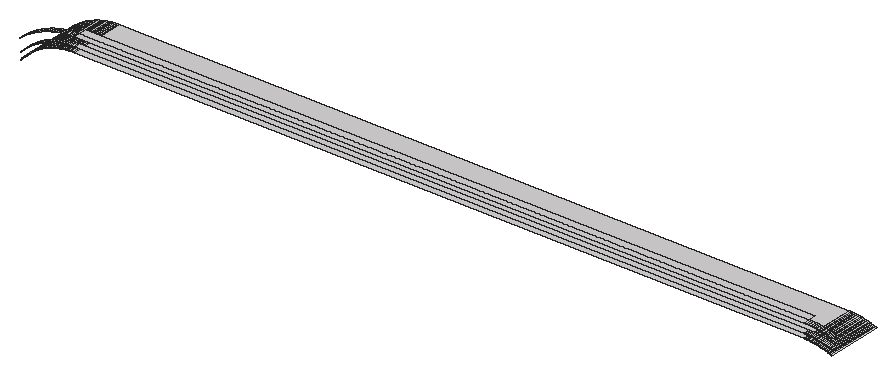
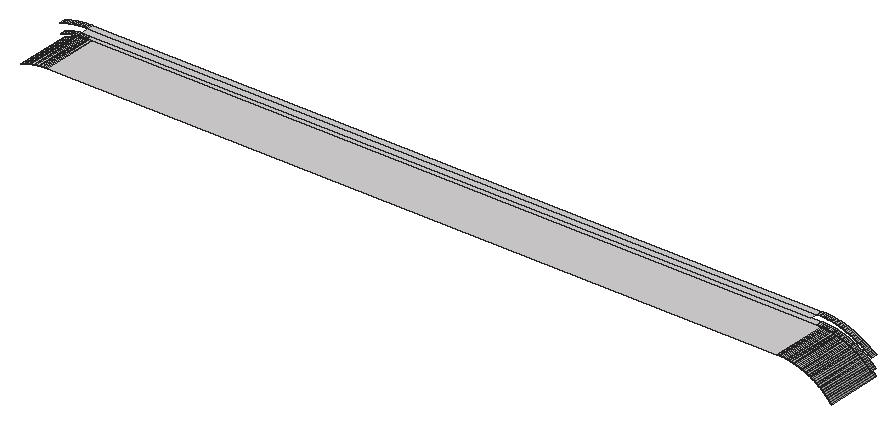
# SketchUp Ruby script. Lengths in inches.
U = 1.inch
M = Sketchup.active_model
def pt(a) = Geom::Point3d.new(a.map { |v| v * U })
def face(e, loops, mat)
  f = e.add_face(loops[0].map { |a| pt(a) })
  loops[1..].each { |l| e.add_face(l.map { |a| pt(a) }).erase! }
  f.material = f.back_material = mat if mat
  f
end
# faces: each face lists its corners as indices into pts; further lists are holes
def faces(e, pts, list, mat = nil) = list.each { |f| face(e, (f[0].is_a?(Array) ? f : [f]).map { |l| l.map { |i| pts[i] } }, mat) }
# xy, xz, yz: faces in a plane at the given z, y or x. An outline is a flat list of corners, or four numbers for a rectangle; further outlines are holes
def ring(l) = l.size == 4 ? [[l[0], l[1]], [l[2], l[1]], [l[2], l[3]], [l[0], l[3]]] : l.each_slice(2).to_a
def flat(e, list, mat, &to3) = list.each { |f| face(e, (f[0].is_a?(Array) ? f : [f]).map { |l| ring(l).map { |u, v| to3.(u, v) } }, mat) }
def xy(e, z, list, mat = nil) = flat(e, list, mat) { |x, y| [x, y, z] }
def xz(e, y, list, mat = nil) = flat(e, list, mat) { |x, z| [x, y, z] }
def yz(e, x, list, mat = nil) = flat(e, list, mat) { |y, z| [x, y, z] }
def lines(e, pts, list) = list.each { |a, b| e.add_line(pt(pts[a]), pt(pts[b])) }
# prism: a flat outline (further loops are holes) pulled along v
def prism(e, loops, v, mat = nil)
  f = face(e, loops, mat); d = Geom::Vector3d.new(v.map { |x| x * U })
  f.pushpull(f.normal.samedirection?(d) ? d.length : -d.length)
end
def box(e, o, s, mat = nil) = prism(e, [[o, [o[0] + s[0], o[1], o[2]], [o[0] + s[0], o[1] + s[1], o[2]], [o[0], o[1] + s[1], o[2]]]], [0, 0, s[2]], mat)
def at(x, y, z, deg = 0) = Geom::Transformation.translation(pt([x, y, z])) * Geom::Transformation.rotation(ORIGIN, Z_AXIS, deg.degrees)
def axes(o, x, y, z) = Geom::Transformation.new([*x, 0, *y, 0, *z, 0, *pt(o).to_a, 1])
def part(name) = M.definitions.add(name)
# library, detail: a bought-in or finely detailed component or shape, given as its bounding box
def library(name, o, s) = part(name).tap { |d| box(d.entities, o, s) }
def detail(e, o, s) = box(e.add_group.entities, o, s)
def put(e, d, t, mat = nil) = e.add_instance(d, t).tap { |i| i.material = mat if mat }
def group(e, t, mat = nil) = e.add_group.tap { |g| g.transformation = t; g.material = mat if mat }.entities
root = M.entities
M.materials.add("[Quartz Light Brown]").color = [215, 212, 212]
xy(root,350.99,[[292.91,143,293.11,155],[450.39,143,450.59,155]],"[Quartz Light Brown]")
xy(root,351,[[293.3,143,293.5,155],[293.5,143,450,155],[450,143,450.2,155]],"[Quartz Light Brown]")
xy(root,351.99,[[292.87,143,293.08,144.25],[450.42,143,450.63,144.25]],"[Quartz Light Brown]")
xy(root,352,[[293.29,143,293.5,144.25],[293.5,143,450,144.25],[450,143,450.21,144.25]],"[Quartz Light Brown]")
xy(root,353.99,[[292.79,143,293.03,144.25],[450.47,143,450.71,144.25]],"[Quartz Light Brown]")
xy(root,354,[[293.26,143,293.5,144.25],[293.5,143,450,144.25],[450,143,450.24,144.25],[293.5,144.25,450,146]],"[Quartz Light Brown]")
p = [[281.97,143,345.59],[281.84,143,345.44],[281.84,155,345.44],[281.97,155,345.59],[282.09,143,345.74],[282.09,155,345.74],
  [282.22,143,345.89],[282.22,155,345.89],[282.35,143,346.04],[282.35,155,346.04],[282.49,143,346.18],[282.49,155,346.18],
  [282.62,143,346.33],[282.62,155,346.33],[282.76,143,346.47],[282.76,155,346.47],[282.89,143,346.61],[282.89,155,346.61],
  [283.03,143,346.74],[283.03,155,346.74],[283.17,143,346.88],[283.17,155,346.88],[283.32,143,347.01],[283.32,155,347.01],
  [281.89,143,347.01],[282.04,143,347.16],[282.04,144.25,347.16],[281.89,144.25,347.01],[283.46,143,347.15],[283.46,155,347.15],
  [283.61,143,347.28],[283.61,155,347.28],[282.1875,143,347.3125],[282.1875,144.25,347.3125],[282.34,143,347.46],[282.34,144.25,347.46],
  [283.76,143,347.41],[283.76,155,347.41],[283.91,143,347.53],[283.91,155,347.53],[282.49,143,347.61],[282.49,144.25,347.61],
  [284.06,143,347.66],[284.06,155,347.66],[282.64,143,347.75],[282.64,144.25,347.75],[282.79,143,347.89],[282.79,144.25,347.89],
  [284.21,143,347.78],[284.21,155,347.78],[284.37,143,347.9],[284.37,155,347.9],[282.95,143,348.03],[282.95,144.25,348.03],
  [284.53,143,348.02],[284.53,155,348.02],[283.11,143,348.17],[283.11,144.25,348.17],[284.68,143,348.14],[284.68,155,348.14],
  [284.84,143,348.25],[284.84,155,348.25],[283.27,143,348.3],[283.27,144.25,348.3],[285,143,348.36],[285,155,348.36],
  [283.43,143,348.43],[283.43,144.25,348.43],[283.59,143,348.57],[283.59,144.25,348.57],[285.17,143,348.47],[285.17,155,348.47],
  [285.33,143,348.58],[285.33,155,348.58],[283.76,143,348.69],[283.76,144.25,348.69],[285.5,143,348.6875],[285.5,155,348.6875],
  [283.93,143,348.82],[283.93,144.25,348.82],[285.66,143,348.79],[285.66,155,348.79],[284.1,143,348.94],[284.1,144.25,348.94],
  [285.83,143,348.89],[285.83,155,348.89],[284.27,143,349.07],[284.27,144.25,349.07],[286,143,348.99],[286,155,348.99],
  [286.17,143,349.09],[286.17,155,349.09],[284.4375,143,349.1875],[284.4375,144.25,349.1875],[286.34,143,349.18],[286.34,155,349.18],
  [284.61,143,349.3],[284.61,144.25,349.3],[286.52,143,349.27],[286.52,155,349.27],[284.79,143,349.42],[284.79,144.25,349.42],
  [286.69,143,349.37],[286.69,155,349.37],[284.96,143,349.53],[284.96,144.25,349.53],[286.87,143,349.45],[286.87,155,349.45],
  [285.14,143,349.64],[285.14,144.25,349.64],[287.04,143,349.54],[287.04,155,349.54],[287.22,143,349.62],[287.22,155,349.62],
  [285.32,143,349.75],[285.32,144.25,349.75],[287.4,143,349.7],[287.4,155,349.7],[281.99,144.25,349.84],[281.99,143,349.84],
  [281.81,143,349.6875],[281.81,144.25,349.6875],[287.58,143,349.78],[287.58,155,349.78],[282.17,144.25,349.99],[282.17,143,349.99],
  [285.5,143,349.86],[285.5,144.25,349.86],[287.76,143,349.86],[287.76,155,349.86],[455.92,143,349.78],[455.74,143,349.86],
  [455.74,155,349.86],[455.92,155,349.78],[285.68,143,349.96],[285.68,144.25,349.96],[287.94,143,349.93],[287.94,155,349.93],
  [288.125,143,350],[288.125,155,350],[455.56,143,349.93],[455.375,143,350],[455.375,155,350],[455.56,155,349.93],
  [282.36,144.25,350.14],[282.36,143,350.14],[285.87,143,350.0625],[285.87,144.25,350.0625],[288.31,143,350.07],[288.31,155,350.07],
  [455.19,143,350.07],[455.19,155,350.07],[282.54,144.25,350.28],[282.54,143,350.28],[286.05,143,350.16],[286.05,144.25,350.16],
  [288.49,143,350.14],[288.49,155,350.14],[288.68,143,350.2],[288.68,155,350.2],[455.01,143,350.14],[454.82,143,350.2],
  [454.82,155,350.2],[455.01,155,350.14],[286.24,143,350.26],[286.24,144.25,350.26],[288.86,143,350.27],[288.86,155,350.27],
  [454.64,143,350.27],[454.64,155,350.27],[282.73,144.25,350.42],[282.73,143,350.42],[286.42,143,350.35],[286.42,144.25,350.35],
  [286.61,143,350.44],[286.61,144.25,350.44],[289.05,143,350.33],[289.05,155,350.33],[289.24,143,350.38],[289.24,155,350.38],
  [454.45,143,350.33],[454.26,143,350.38],[454.26,155,350.38],[454.45,155,350.33],[282.92,144.25,350.5625],[282.92,143,350.5625],
  [286.8,143,350.53],[286.8,144.25,350.53],[289.43,143,350.4375],[289.43,155,350.4375],[289.62,143,350.49],[289.62,155,350.49],
  [454.07,143,350.4375],[453.88,143,350.49],[453.88,155,350.49],[454.07,155,350.4375],[286.99,143,350.62],[286.99,144.25,350.62],
  [289.81,143,350.54],[289.81,155,350.54],[290,143,350.59],[290,155,350.59],[453.69,143,350.54],[453.5,143,350.59],
  [453.5,155,350.59],[453.69,155,350.54],[283.11,144.25,350.7],[283.11,143,350.7],[287.18,143,350.7],[287.18,144.25,350.7],
  [290.19,143,350.63],[290.19,155,350.63],[290.38,143,350.67],[290.38,155,350.67],[453.31,143,350.63],[453.12,143,350.67],
  [453.12,155,350.67],[453.31,155,350.63],[283.3,144.25,350.83],[283.3,143,350.83],[287.38,143,350.78],[287.38,144.25,350.78],
  [290.57,143,350.71],[290.57,155,350.71],[290.77,143,350.75],[290.77,155,350.75],[290.96,143,350.78],[290.96,155,350.78],
  [452.73,143,350.75],[452.54,143,350.78],[452.54,155,350.78],[452.73,155,350.75],[452.93,143,350.71],[452.93,155,350.71],
  [283.5,144.25,350.97],[283.5,143,350.97],[287.57,143,350.86],[287.57,144.25,350.86],[291.15,143,350.82],[291.15,155,350.82],
  [291.35,143,350.84],[291.35,155,350.84],[291.54,143,350.87],[291.54,155,350.87],[452.15,143,350.84],[451.96,143,350.87],
  [451.96,155,350.87],[452.15,155,350.84],[452.35,143,350.82],[452.35,155,350.82],[287.77,143,350.9375],[287.77,144.25,350.9375],
  [287.96,143,351.01],[287.96,144.25,351.01],[291.74,143,350.9],[291.74,155,350.9],[291.93,143,350.92],[291.93,155,350.92],
  [292.13,143,350.9375],[292.13,155,350.9375],[292.32,143,350.95],[292.32,155,350.95],[451.37,143,350.9375],[451.18,143,350.95],
  [451.18,155,350.95],[451.37,155,350.9375],[451.57,143,350.92],[451.57,155,350.92],[451.76,143,350.9],[451.76,155,350.9],
  [455.54,143,351.01],[455.73,143,350.9375],[455.73,144.25,350.9375],[455.54,144.25,351.01],[455.93,143,350.86],[455.93,144.25,350.86],
  [283.7,144.25,351.1],[283.7,143,351.1],[288.16,143,351.08],[288.16,144.25,351.08],[292.52,143,350.97],[292.52,155,350.97],
  [292.71,143,350.98],[292.71,155,350.98],[292.91,143,350.99],[292.91,155,350.99],[293.3,143,351],[293.11,143,350.99],
  [293.11,155,350.99],[293.3,155,351],[450.39,143,350.99],[450.2,143,351],[450.2,155,351],[450.39,155,350.99],
  [450.79,143,350.98],[450.59,143,350.99],[450.59,155,350.99],[450.79,155,350.98],[450.98,143,350.97],[450.98,155,350.97],
  [455.34,143,351.08],[455.34,144.25,351.08],[283.89,144.25,351.22],[283.89,143,351.22],[288.36,143,351.15],[288.36,144.25,351.15],
  [455.14,143,351.15],[455.14,144.25,351.15],[284.1,144.25,351.35],[284.1,143,351.35],[288.56,143,351.22],[288.56,144.25,351.22],
  [288.76,143,351.28],[288.76,144.25,351.28],[454.74,143,351.28],[454.94,143,351.22],[454.94,144.25,351.22],[454.74,144.25,351.28],
  [284.3,144.25,351.47],[284.3,143,351.47],[288.96,143,351.34],[288.96,144.25,351.34],[289.16,143,351.4],[289.16,144.25,351.4],
  [454.34,143,351.4],[454.54,143,351.34],[454.54,144.25,351.34],[454.34,144.25,351.4],[289.36,143,351.45],[289.36,144.25,351.45],
  [454.14,143,351.45],[454.14,144.25,351.45],[284.5,144.25,351.59],[284.5,143,351.59],[289.5625,143,351.51],[289.5625,144.25,351.51],
  [289.76,143,351.56],[289.76,144.25,351.56],[453.74,143,351.56],[453.9375,143,351.51],[453.9375,144.25,351.51],[453.74,144.25,351.56],
  [284.7,144.25,351.7],[284.7,143,351.7],[289.97,143,351.61],[289.97,144.25,351.61],[290.17,143,351.65],[290.17,144.25,351.65],
  [453.33,143,351.65],[453.53,143,351.61],[453.53,144.25,351.61],[453.33,144.25,351.65],[284.91,144.25,351.82],[284.91,143,351.82],
  [290.38,143,351.69],[290.38,144.25,351.69],[290.58,143,351.73],[290.58,144.25,351.73],[290.79,143,351.77],[290.79,144.25,351.77],
  [452.71,143,351.77],[452.92,143,351.73],[452.92,144.25,351.73],[452.71,144.25,351.77],[453.12,143,351.69],[453.12,144.25,351.69],
  [285.12,144.25,351.93],[285.12,143,351.93],[291,143,351.8],[291,144.25,351.8],[291.2,143,351.83],[291.2,144.25,351.83],
  [291.41,143,351.86],[291.41,144.25,351.86],[452.09,143,351.86],[452.3,143,351.83],[452.3,144.25,351.83],[452.09,144.25,351.86],
  [452.5,143,351.8],[452.5,144.25,351.8],[285.33,144.25,352.04],[285.33,143,352.04],[291.62,143,351.89],[291.62,144.25,351.89],
  [291.83,143,351.91],[291.83,144.25,351.91],[292.04,143,351.93],[292.04,144.25,351.93],[292.24,143,351.95],[292.24,144.25,351.95],
  [451.26,143,351.95],[451.46,143,351.93],[451.46,144.25,351.93],[451.26,144.25,351.95],[451.67,143,351.91],[451.67,144.25,351.91],
  [451.88,143,351.89],[451.88,144.25,351.89],[285.54,144.25,352.14],[285.54,143,352.14],[292.45,143,351.97],[292.45,144.25,351.97],
  [292.66,143,351.98],[292.66,144.25,351.98],[292.87,143,351.99],[292.87,144.25,351.99],[293.08,143,351.99],[293.29,143,352],
  [293.29,144.25,352],[293.08,144.25,351.99],[450.21,143,352],[450.42,143,351.99],[450.42,144.25,351.99],[450.21,144.25,352],
  [450.63,143,351.99],[450.84,143,351.98],[450.84,144.25,351.98],[450.63,144.25,351.99],[451.05,143,351.97],[451.05,144.25,351.97],
  [285.75,144.25,352.25],[285.75,143,352.25],[285.96,144.25,352.35],[285.96,143,352.35],[286.18,144.25,352.44],[286.18,143,352.44],
  [286.39,144.25,352.54],[286.39,143,352.54],[286.61,144.25,352.63],[286.61,143,352.63],[286.83,144.25,352.72],[286.83,143,352.72],
  [287.05,144.25,352.8],[287.05,143,352.8],[287.27,144.25,352.89],[287.27,143,352.89],[287.49,144.25,352.97],[287.49,143,352.97],
  [287.71,144.25,353.04],[287.71,143,353.04],[287.9375,144.25,353.12],[287.9375,143,353.12],[455.79,144.25,353.04],[455.79,143,353.04],
  [455.5625,143,353.12],[455.5625,144.25,353.12],[456.01,144.25,352.97],[456.01,143,352.97],[288.16,144.25,353.19],[288.16,143,353.19],
  [455.34,143,353.19],[455.34,144.25,353.19],[288.39,144.25,353.26],[288.39,143,353.26],[455.11,143,353.26],[455.11,144.25,353.26],
  [288.61,144.25,353.32],[288.61,143,353.32],[288.84,144.25,353.39],[288.84,143,353.39],[454.89,144.25,353.32],[454.89,143,353.32],
  [454.66,143,353.39],[454.66,144.25,353.39],[289.07,144.25,353.45],[289.07,143,353.45],[289.3,144.25,353.5],[289.3,143,353.5],
  [454.43,144.25,353.45],[454.43,143,353.45],[454.2,143,353.5],[454.2,144.25,353.5],[289.53,144.25,353.56],[289.53,143,353.56],
  [453.97,143,353.56],[453.97,144.25,353.56],[289.76,144.25,353.61],[289.76,143,353.61],[289.99,144.25,353.65],[289.99,143,353.65],
  [453.74,144.25,353.61],[453.74,143,353.61],[453.51,143,353.65],[453.51,144.25,353.65],[290.22,144.25,353.7],[290.22,143,353.7],
  [290.45,144.25,353.74],[290.45,143,353.74],[290.68,144.25,353.78],[290.68,143,353.78],[453.05,144.25,353.74],[453.05,143,353.74],
  [452.82,143,353.78],[452.82,144.25,353.78],[453.28,144.25,353.7],[453.28,143,353.7],[290.92,144.25,353.8125],[290.92,143,353.8125],
  [291.15,144.25,353.85],[291.15,143,353.85],[291.38,144.25,353.875],[291.38,143,353.875],[452.35,144.25,353.85],[452.35,143,353.85],
  [452.12,143,353.875],[452.12,144.25,353.875],[452.58,144.25,353.8125],[452.58,143,353.8125],[291.62,144.25,353.9],[291.62,143,353.9],
  [291.85,144.25,353.92],[291.85,143,353.92],[292.09,144.25,353.94],[292.09,143,353.94],[292.32,144.25,353.96],[292.32,143,353.96],
  [451.41,144.25,353.94],[451.41,143,353.94],[451.18,143,353.96],[451.18,144.25,353.96],[451.65,144.25,353.92],[451.65,143,353.92],
  [451.88,144.25,353.9],[451.88,143,353.9],[292.56,144.25,353.98],[292.56,143,353.98],[292.79,144.25,353.99],[292.79,143,353.99],
  [293.26,144.25,354],[293.26,143,354],[293.03,143,353.99],[293.03,144.25,353.99],[450.47,144.25,353.99],[450.47,143,353.99],
  [450.24,143,354],[450.24,144.25,354],[450.94,144.25,353.98],[450.94,143,353.98],[450.71,143,353.99],[450.71,144.25,353.99]]
faces(root,p,[[0,1,2,3],[4,0,3,5],[6,4,5,7],[8,6,7,9],[10,8,9,11],[12,10,11,13],[14,12,13,15],[16,14,15,17],
  [18,16,17,19],[20,18,19,21],[22,20,21,23],[24,25,26,27],[28,22,23,29],[30,28,29,31],[25,32,33,26],[32,34,35,33],
  [36,30,31,37],[38,36,37,39],[34,40,41,35],[42,38,39,43],[40,44,45,41],[44,46,47,45],[48,42,43,49],[50,48,49,51],
  [46,52,53,47],[54,50,51,55],[52,56,57,53],[58,54,55,59],[60,58,59,61],[56,62,63,57],[64,60,61,65],[62,66,67,63],
  [66,68,69,67],[70,64,65,71],[72,70,71,73],[68,74,75,69],[76,72,73,77],[74,78,79,75],[80,76,77,81],[78,82,83,79],
  [84,80,81,85],[82,86,87,83],[88,84,85,89],[90,88,89,91],[86,92,93,87],[94,90,91,95],[92,96,97,93],[98,94,95,99],
  [96,100,101,97],[102,98,99,103],[100,104,105,101],[106,102,103,107],[104,108,109,105],[110,106,107,111],[112,110,111,113],[108,114,115,109],
  [116,112,113,117],[118,119,120,121],[122,116,117,123],[124,125,119,118],[114,126,127,115],[128,122,123,129],[130,131,132,133],[126,134,135,127],
  [136,128,129,137],[138,136,137,139],[140,141,142,143],[131,140,143,132],[144,145,125,124],[134,146,147,135],[148,138,139,149],[141,150,151,142],
  [152,153,145,144],[146,154,155,147],[156,148,149,157],[158,156,157,159],[160,161,162,163],[150,160,163,151],[154,164,165,155],[166,158,159,167],
  [161,168,169,162],[170,171,153,152],[164,172,173,165],[172,174,175,173],[176,166,167,177],[178,176,177,179],[180,181,182,183],[168,180,183,169],
  [184,185,171,170],[174,186,187,175],[188,178,179,189],[190,188,189,191],[192,193,194,195],[181,192,195,182],[186,196,197,187],[198,190,191,199],
  [200,198,199,201],[202,203,204,205],[193,202,205,194],[206,207,185,184],[196,208,209,197],[210,200,201,211],[212,210,211,213],[214,215,216,217],
  [203,214,217,204],[218,219,207,206],[208,220,221,209],[222,212,213,223],[224,222,223,225],[226,224,225,227],[228,229,230,231],[232,228,231,233],
  [215,232,233,216],[234,235,219,218],[220,236,237,221],[238,226,227,239],[240,238,239,241],[242,240,241,243],[244,245,246,247],[248,244,247,249],
  [229,248,249,230],[236,250,251,237],[250,252,253,251],[254,242,243,255],[256,254,255,257],[258,256,257,259],[260,258,259,261],[262,263,264,265],
  [266,262,265,267],[268,266,267,269],[245,268,269,246],[270,271,272,273],[271,274,275,272],[276,277,235,234],[252,278,279,253],[280,260,261,281],
  [282,280,281,283],[284,282,283,285],[286,287,288,289],[290,291,292,293],[294,295,296,297],[298,294,297,299],[263,298,299,264],[300,270,273,301],
  [302,303,277,276],[278,304,305,279],[306,300,301,307],[308,309,303,302],[304,310,311,305],[310,312,313,311],[314,315,316,317],[315,306,307,316],
  [318,319,309,308],[312,320,321,313],[320,322,323,321],[324,325,326,327],[325,314,317,326],[322,328,329,323],[330,324,327,331],[332,333,319,318],
  [328,334,335,329],[334,336,337,335],[338,339,340,341],[339,330,331,340],[342,343,333,332],[336,344,345,337],[344,346,347,345],[348,349,350,351],
  [349,338,341,350],[352,353,343,342],[346,354,355,347],[354,356,357,355],[356,358,359,357],[360,361,362,363],[361,364,365,362],[364,348,351,365],
  [366,367,353,352],[358,368,369,359],[368,370,371,369],[370,372,373,371],[374,375,376,377],[375,378,379,376],[378,360,363,379],[380,381,367,366],
  [372,382,383,373],[382,384,385,383],[384,386,387,385],[386,388,389,387],[390,391,392,393],[391,394,395,392],[394,396,397,395],[396,374,377,397],
  [398,399,381,380],[388,400,401,389],[400,402,403,401],[402,404,405,403],[406,407,408,409],[410,411,412,413],[414,415,416,417],[415,418,419,416],
  [418,390,393,419],[420,421,399,398],[422,423,421,420],[424,425,423,422],[426,427,425,424],[428,429,427,426],[430,431,429,428],[432,433,431,430],
  [434,435,433,432],[436,437,435,434],[438,439,437,436],[440,441,439,438],[442,443,444,445],[446,447,443,442],[448,449,441,440],[445,444,450,451],
  [452,453,449,448],[451,450,454,455],[456,457,453,452],[458,459,457,456],[460,461,462,463],[455,454,461,460],[464,465,459,458],[466,467,465,464],
  [468,469,470,471],[463,462,469,468],[472,473,467,466],[471,470,474,475],[476,477,473,472],[478,479,477,476],[480,481,482,483],[475,474,481,480],
  [484,485,479,478],[486,487,485,484],[488,489,487,486],[490,491,492,493],[494,495,491,490],[483,482,495,494],[496,497,489,488],[498,499,497,496],
  [500,501,499,498],[502,503,504,505],[506,507,503,502],[493,492,507,506],[508,509,501,500],[510,511,509,508],[512,513,511,510],[514,515,513,512],
  [516,517,518,519],[520,521,517,516],[522,523,521,520],[505,504,523,522],[524,525,515,514],[526,527,525,524],[528,529,530,531],[532,533,534,535],
  [536,537,538,539],[519,518,537,536]],"[Quartz Light Brown]")
